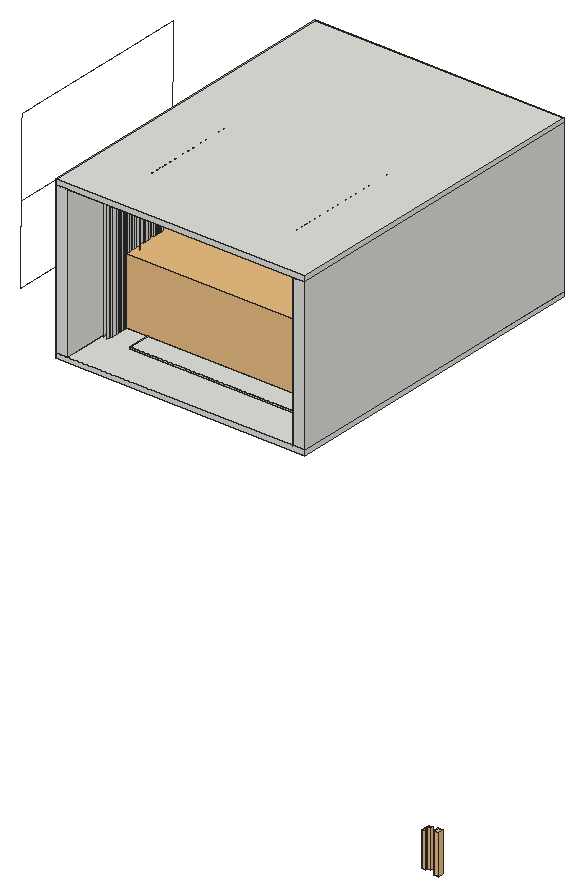
# SketchUp Ruby script. Lengths in millimetres.
U = 1.mm
M = Sketchup.active_model
def pt(a) = Geom::Point3d.new(a.map { |v| v * U })
def face(e, loops, mat)
  f = e.add_face(loops[0].map { |a| pt(a) })
  loops[1..].each { |l| e.add_face(l.map { |a| pt(a) }).erase! }
  f.material = f.back_material = mat if mat
  f
end
# faces: each face lists its corners as indices into pts; further lists are holes
def faces(e, pts, list, mat = nil) = list.each { |f| face(e, (f[0].is_a?(Array) ? f : [f]).map { |l| l.map { |i| pts[i] } }, mat) }
# xy, xz, yz: faces in a plane at the given z, y or x. An outline is a flat list of corners, or four numbers for a rectangle; further outlines are holes
def ring(l) = l.size == 4 ? [[l[0], l[1]], [l[2], l[1]], [l[2], l[3]], [l[0], l[3]]] : l.each_slice(2).to_a
def flat(e, list, mat, &to3) = list.each { |f| face(e, (f[0].is_a?(Array) ? f : [f]).map { |l| ring(l).map { |u, v| to3.(u, v) } }, mat) }
def xy(e, z, list, mat = nil) = flat(e, list, mat) { |x, y| [x, y, z] }
def xz(e, y, list, mat = nil) = flat(e, list, mat) { |x, z| [x, y, z] }
def yz(e, x, list, mat = nil) = flat(e, list, mat) { |y, z| [x, y, z] }
def lines(e, pts, list) = list.each { |a, b| e.add_line(pt(pts[a]), pt(pts[b])) }
# prism: a flat outline (further loops are holes) pulled along v
def prism(e, loops, v, mat = nil)
  f = face(e, loops, mat); d = Geom::Vector3d.new(v.map { |x| x * U })
  f.pushpull(f.normal.samedirection?(d) ? d.length : -d.length)
end
def box(e, o, s, mat = nil) = prism(e, [[o, [o[0] + s[0], o[1], o[2]], [o[0] + s[0], o[1] + s[1], o[2]], [o[0], o[1] + s[1], o[2]]]], [0, 0, s[2]], mat)
def at(x, y, z, deg = 0) = Geom::Transformation.translation(pt([x, y, z])) * Geom::Transformation.rotation(ORIGIN, Z_AXIS, deg.degrees)
def axes(o, x, y, z) = Geom::Transformation.new([*x, 0, *y, 0, *z, 0, *pt(o).to_a, 1])
def part(name) = M.definitions.add(name)
# library, detail: a bought-in or finely detailed component or shape, given as its bounding box
def library(name, o, s) = part(name).tap { |d| box(d.entities, o, s) }
def detail(e, o, s) = box(e.add_group.entities, o, s)
def put(e, d, t, mat = nil) = e.add_instance(d, t).tap { |i| i.material = mat if mat }
def group(e, t, mat = nil) = e.add_group.tap { |g| g.transformation = t; g.material = mat if mat }.entities
root = M.entities
M.materials.add("Glass").color = [171, 209, 242]
M.materials["Glass"].alpha = 0.1
M.materials.add("Plastic_SSS_01_White").color = [225, 221, 201]
M.materials.add("[0136_Charcoal]").color = [35, 35, 35]
M.materials.add("[Color A08]").color = [102, 0, 0]
M.materials.add("[Color M07]").color = [58, 58, 58]
M.materials.add("[Formica Beige]").color = [211, 187, 149]
M.materials.add("[Wood Veneer 01]").color = [120, 70, 37]
M.materials.add("тюль").color = [255, 255, 255]
M.materials["тюль"].alpha = 0.6
c1 = part("Area rug")
box(c1.entities,[0,0,0],[1400,2000,10])
c2 = part("Window frame")
xy(c2.entities,0,[[[2653.4,2133.1,4482.2,3352.3],[2704.2,2183.9,4431.4,3301.5]],[3237.6,2183.9,3288.4,3301.5],[3821.8,2183.9,3872.6,3301.5]],"Plastic_SSS_01_White")
xy(c2.entities,50.8,[[[2653.4,2133.1,4482.2,3352.3],[2704.2,2183.9,4431.4,3301.5]],[3237.6,2183.9,3288.4,3301.5],[3821.8,2183.9,3872.6,3301.5]],"Plastic_SSS_01_White")
xz(c2.entities,2133.1,[[2653.4,0,4482.2,50.8]],"Plastic_SSS_01_White")
xz(c2.entities,2183.9,[[2704.2,0,3237.6,50.8],[3237.6,0,3288.4,50.8],[3288.4,0,3821.8,50.8],[3821.8,0,3872.6,50.8],[3872.6,0,4431.4,50.8]],"Plastic_SSS_01_White")
xz(c2.entities,3301.5,[[2704.2,0,3237.6,50.8],[3237.6,0,3288.4,50.8],[3288.4,0,3821.8,50.8],[3821.8,0,3872.6,50.8],[3872.6,0,4431.4,50.8]],"Plastic_SSS_01_White")
xz(c2.entities,3352.3,[[2653.4,0,4482.2,50.8]],"Plastic_SSS_01_White")
yz(c2.entities,2653.4,[[2133.1,0,3352.3,50.8]],"Plastic_SSS_01_White")
yz(c2.entities,2704.2,[[2183.9,0,3301.5,50.8]],"Plastic_SSS_01_White")
yz(c2.entities,3237.6,[[2183.9,0,3301.5,50.8]],"Plastic_SSS_01_White")
yz(c2.entities,3288.4,[[2183.9,0,3301.5,50.8]],"Plastic_SSS_01_White")
yz(c2.entities,3821.8,[[2183.9,0,3301.5,50.8]],"Plastic_SSS_01_White")
yz(c2.entities,3872.6,[[2183.9,0,3301.5,50.8]],"Plastic_SSS_01_White")
yz(c2.entities,4431.4,[[2183.9,0,3301.5,50.8]],"Plastic_SSS_01_White")
yz(c2.entities,4482.2,[[2133.1,0,3352.3,50.8]],"Plastic_SSS_01_White")
c3 = part("Window glazing")
box(c3.entities,[0,0,0],[1724.1,1117.6,12.7])
c4 = part("Window assembly")
put(c4.entities,c2,at(-2653.4,-2133.1,0))
put(c4.entities,c3,at(50.8,50.8,17.8),"Glass")
c5 = part("window")
p = [[-15145.6,2238.1,518],[-16974.4,2238.1,518]]
lines(c5.entities,p,[[0,1]])
put(c5.entities,c4,axes([-16974.4,2238.1,518],[1,0,0],[0,0,1],[0,-1,0]))
c6 = part("Group\#61")
p = [[0,48,9.6],[0,48,40.8],[0,18.3,0],[0,0,25.2],[0,18.3,50.4]]
lines(c6.entities,p,[[0,1],[2,0],[3,2],[4,3],[1,4]])
c7 = part("Curtain panel")
yz(c7.entities,423.5,[[83.6,68.6,120.5,2032]])
p = [[42.2,57.1,68.6],[81.9,49.1,68.6],[81.9,49.1,2032],[42.2,57.1,2032],[89.6,60.6,68.6],[89.6,60.6,2032],
  [250.5,51.4,68.6],[262,49.4,68.6],[262,49.4,2032],[250.5,51.4,2032],[294,52.7,68.6],[294,52.7,2032],
  [234.4,66.2,68.6],[234.4,66.2,2032],[335.4,52.5,68.6],[351.9,52.1,68.6],[351.9,52.1,2032],[335.4,52.5,2032],
  [375.5,60,68.6],[375.5,60,2032],[332,60.7,68.6],[332,60.7,2032],[302.6,99.4,68.6],[302.6,99.4,2032],
  [113.7,56.1,68.6],[116.9,54,68.6],[116.9,54,2032],[113.7,56.1,2032],[130.3,54.1,68.6],[130.3,54.1,2032],
  [142.4,61.5,68.6],[142.4,61.5,2032],[485.4,55.1,68.6],[498.9,54.2,68.6],[498.9,54.2,2032],[485.4,55.1,2032],
  [509.2,55.8,2032],[509.2,55.8,68.6],[479.1,58.2,68.6],[479.1,58.2,2032],[168.4,60.1,68.6],[183.1,55.5,68.6],
  [183.1,55.5,2032],[168.4,60.1,2032],[205.8,56.2,68.6],[205.8,56.2,2032],[106,65.3,68.6],[106,65.3,2032],
  [220.7,98.3,68.6],[220.7,98.3,2032],[18.5,73.5,68.6],[18.5,73.5,2032],[475.8,65.4,68.6],[475.8,65.4,2032],
  [438.7,58.9,68.6],[448,58.5,68.6],[448,58.5,2032],[438.7,58.9,2032],[452.1,62.6,68.6],[452.1,62.6,2032],
  [428.3,61.4,68.6],[428.3,61.4,2032],[387.2,83.9,68.6],[387.2,83.9,2032],[165,66.8,68.6],[165,66.8,2032],
  [72.3,95.7,68.6],[72.3,95.7,2032],[343.3,92.9,68.6],[343.3,92.9,2032],[425,65.5,68.6],[425,65.5,2032],
  [156.5,93.7,68.6],[156.5,93.7,2032],[442.7,100.9,68.6],[442.7,100.9,2032],[100.8,87.1,68.6],[100.8,87.1,2032],
  [474.1,91.8,68.6],[474.1,91.8,2032],[423.5,83.6,68.6],[423.5,83.6,2032],[235.7,85.9,68.6],[235.7,85.9,2032],
  [190.8,117.3,68.6],[190.8,117.3,2032],[24.1,85.5,68.6],[24.1,85.5,2032],[379.7,124.4,68.6],[379.7,124.4,2032],
  [35.1,112.6,68.6],[35.1,112.6,2032],[267.2,131.4,68.6],[267.2,131.4,2032],[112,135,68.6],[112,135,2032],
  [486.8,123.6,68.6],[486.8,123.6,2032],[346.6,120.5,68.6],[346.6,120.5,2032],[152.9,128.5,68.6],[152.9,128.5,2032],
  [56.6,138.8,68.6],[56.6,138.8,2032],[221.5,129.5,68.6],[221.5,129.5,2032],[301.6,129,68.6],[301.6,129,2032],
  [432.5,131,68.6],[432.5,131,2032],[24,125.5,68.6],[24,125.5,2032],[173.3,137,68.6],[173.3,137,2032],
  [330.4,136,68.6],[330.4,136,2032],[409.6,134,68.6],[423.5,120.5,68.6],[423.5,120.5,2032],[409.6,134,2032],
  [473.8,143.8,68.6],[473.8,143.8,2032],[388.8,133.8,68.6],[388.8,133.8,2032],[0,139.4,68.6],[0,139.4,2032],
  [236.4,146.3,68.6],[236.4,146.3,2032],[439.5,142.5,2032],[439.5,142.5,68.6],[266.8,141.8,68.6],[266.8,141.8,2032],
  [101,147.4,68.6],[101,147.4,2032],[519.5,57.4,2032],[527.7,61.1,2032]]
faces(c7.entities,p,[[0,1,2,3],[1,4,5,2],[6,7,8,9],[7,10,11,8],[12,6,9,13],[14,15,16,17],[15,18,19,16],[20,14,17,21],
  [10,22,23,11],[24,25,26,27],[25,28,29,26],[28,30,31,29],[32,33,34,35],[36,34,33,37],[38,32,35,39],[40,41,42,43],
  [41,44,45,42],[46,24,27,47],[44,48,49,45],[50,0,3,51],[52,38,39,53],[54,55,56,57],[55,58,59,56],[60,54,57,61],
  [18,62,63,19],[64,40,43,65],[4,66,67,5],[68,20,21,69],[70,60,61,71],[30,72,73,31],[58,74,75,59],[76,46,47,77],
  [78,52,53,79],[80,70,71,81],[82,12,13,83],[84,64,65,85],[86,50,51,87],[62,88,89,63],[90,86,87,91],[92,82,83,93],
  [94,76,77,95],[96,78,79,97],[98,68,69,99],[72,100,101,73],[66,102,103,67],[48,104,105,49],[22,106,107,23],[74,108,109,75],
  [110,90,91,111],[112,84,85,113],[114,98,99,115],[116,117,118,119],[120,96,97,121],[88,122,123,89],[124,110,111,125],[100,112,113,101],
  [106,114,115,107],[104,126,127,105],[128,109,108,129],[130,92,93,131],[122,116,119,123],[132,94,95,133],[102,132,133,103],[126,130,131,127],
  [129,120,121,128]])
lines(c7.entities,p,[[134,135]])
put(c7.entities,c6,at(248.1,127.4,2032,-180))
put(c7.entities,c6,at(302.6,127.4,2032,-180))
put(c7.entities,c6,at(344,127.4,2032,-180))
put(c7.entities,c6,at(185.2,127.4,2032,-180))
put(c7.entities,c6,at(157,127.4,2032,-180))
put(c7.entities,c6,at(220.8,127.4,2032,-180))
put(c7.entities,c6,at(442.4,128,2032,-180))
put(c7.entities,c6,at(479,128,2032,-180))
put(c7.entities,c6,at(383.2,127.4,2032,-180))
put(c7.entities,c6,at(423.2,128,2032,-180))
put(c7.entities,c6,at(64.5,127.4,2032,-180))
put(c7.entities,c6,at(35.1,127.4,2032,-180))
put(c7.entities,c6,at(104.2,127.4,2032,-180))
c8 = part("end")
yz(c8.entities,0,[[32.5,25.8,24.5,28.4,24.5,36.8,32.5,39.4,37.5,32.6]])
p = [[50.8,0,12.5],[0,24.5,28.4],[0,32.5,25.8],[50.8,38.3,0],[101.6,13.8,21.4],[101.6,35.1,14.5],
  [0,37.5,32.6],[50.8,62,32.6],[101.6,48.2,32.6],[50.8,0,52.8],[0,24.5,36.8],[101.6,13.8,43.8],
  [0,32.5,39.4],[50.8,38.3,65.2],[101.6,35.1,50.7]]
faces(c8.entities,p,[[0,1,2,3],[4,0,3,5],[3,2,6,7],[3,7,8,5],[0,9,10,1],[4,11,9,0],[6,12,13,7],[7,13,14,8],
  [13,12,10,9],[14,13,9,11]])
c9 = part("Component\#75")
p = [[0,51.3,30.2],[0,25.7,48.8],[0,41.5,0],[0,0,30.2],[0,9.8,0]]
lines(c9.entities,p,[[0,1],[2,0],[3,4],[4,2],[1,3]])
c10 = part("Shower curtain\#1")
xy(c10.entities,-12.7,[[707,-12.7,2483.6,0]],"[0136_Charcoal]")
xy(c10.entities,0,[[707,-12.7,2483.6,0]],"[0136_Charcoal]")
xz(c10.entities,-12.7,[[707,-12.7,2483.6,0]],"[0136_Charcoal]")
xz(c10.entities,0,[[707,-12.7,2483.6,0]],"[0136_Charcoal]")
yz(c10.entities,707,[[-12.7,-12.7,0,0]])
yz(c10.entities,2483.6,[[-12.7,-12.7,0,0]],"[0136_Charcoal]")
put(c10.entities,c9,at(413.5,-33.6,-42.9))
put(c10.entities,c9,at(308,-33.6,-42.9))
put(c10.entities,c9,at(637.2,-33.6,-42.9))
put(c10.entities,c9,at(194.5,-33.6,-42.9))
put(c10.entities,c9,at(941,-33.6,-42.9))
put(c10.entities,c9,at(1223.4,-33.6,-42.9))
put(c10.entities,c9,at(761.7,-33.6,-42.9))
put(c10.entities,c9,at(875.2,-33.6,-42.9))
put(c10.entities,c9,at(1478.1,-33.6,-42.9))
put(c10.entities,c9,at(1328.9,-33.6,-42.9))
put(c10.entities,c9,at(81.1,-33.6,-42.9))
put(c10.entities,c9,at(534.9,-33.6,-42.9))
put(c10.entities,c9,at(1102,-33.6,-42.9))
g1 = group(c10.entities,at(18,-33,-2645.8))
p = [[684.3,109.4,0],[523.1,134.5,2.6],[523.1,25.1,2608.1],[684.3,0,2605.5],[803.4,168,6],[803.4,58.6,2611.6],
  [1212,109.4,0],[1177,123.4,1.4],[1177,14,2607],[1212,0,2605.5],[378.3,117.8,0.9],[322.3,156.9,4.9],
  [322.3,47.4,2610.4],[378.3,8.4,2606.4],[91.1,148.5,4],[0,123.4,1.4],[0,14,2607],[91.1,39.1,2609.6],
  [1153.7,148.5,4],[1153.7,39.1,2609.6],[175.2,126.2,1.7],[175.2,16.7,2607.3],[1008.9,131.7,2.3],[903.8,142.9,3.5],
  [903.8,33.5,2609],[1008.9,22.3,2607.8],[885.1,154.1,4.6],[885.1,44.7,2610.1]]
faces(g1,p,[[0,1,2,3],[4,0,3,5],[6,7,8,9],[10,11,12,13],[1,10,13,2],[14,15,16,17],[7,18,19,8],[20,14,17,21],
  [11,20,21,12],[22,23,24,25],[18,22,25,19],[23,26,27,24],[26,4,5,27]],"тюль")
g2 = group(c10.entities,at(1275.1,-33,-2645.8))
p = [[684.3,109.4,0],[523.1,134.5,2.6],[523.1,25.1,2608.1],[684.3,0,2605.5],[803.4,168,6],[803.4,58.6,2611.6],
  [1212,109.4,0],[1177,123.4,1.4],[1177,14,2607],[1212,0,2605.5],[378.3,117.8,0.9],[322.3,156.9,4.9],
  [322.3,47.4,2610.4],[378.3,8.4,2606.4],[91.1,148.5,4],[0,123.4,1.4],[0,14,2607],[91.1,39.1,2609.6],
  [1153.7,148.5,4],[1153.7,39.1,2609.6],[175.2,126.2,1.7],[175.2,16.7,2607.3],[1008.9,131.7,2.3],[903.8,142.9,3.5],
  [903.8,33.5,2609],[1008.9,22.3,2607.8],[885.1,154.1,4.6],[885.1,44.7,2610.1]]
faces(g2,p,[[0,1,2,3],[4,0,3,5],[6,7,8,9],[10,11,12,13],[1,10,13,2],[14,15,16,17],[7,18,19,8],[20,14,17,21],
  [11,20,21,12],[22,23,24,25],[18,22,25,19],[23,26,27,24],[26,4,5,27]],"тюль")
c11 = part("Группа\#112")
xy(c11.entities,34.5,[[707,9,2507,38]],"[0136_Charcoal]")
p = [[2507,23.5,0],[2507,0,13.2],[707,0,13.2],[707,23.5,0],[2507,47,13.2],[707,47,13.2],
  [2507,9,34.5],[707,9,34.5],[2507,38,34.5],[707,38,34.5]]
faces(c11.entities,p,[[0,1,2,3],[4,0,3,5],[1,6,7,2],[8,4,5,9]],"[0136_Charcoal]")
c12 = part("шторы раздвинутые\#1")
put(c12.entities,c7,axes([706.9,-2079.9,174.7],[1,0,0],[0,0,-0.36],[0,1,0]))
put(c12.entities,c7,axes([2242.4,-2079.9,174.7],[-1,0,0],[0,0,-0.36],[0,1,0]))
put(c12.entities,c8,axes([601.7,-53.1,137.5],[1,0,0],[0,0,-1],[0,1,0]),"[0136_Charcoal]")
put(c12.entities,c8,axes([2336.8,-53.1,137.5],[-1,0,0],[0,0,-1],[0,1,0]),"[0136_Charcoal]")
put(c12.entities,c10,axes([695.8,-38.1,43.6],[0.62018,0,0],[0,-0.03238,-0.99912],[0,0.7459,-0.04059]))
put(c12.entities,c11,axes([101.6,-38.6,89.2],[0.85105,0,0],[0,0.77173,0],[0,0,1]))
c13 = library("Кровать",[-199.4,-668.7,0],[2314.3,3237.4,1077.7])
c14 = part("Group103\#1")
p = [[0,0,0],[0,0,-1085.9],[-296.1,0,-1085.9],[1927.9,-1587.5,0],[-1927.9,-1587.5,0],[1927.9,1587.5,0],
  [1927.9,0,0],[-1927.9,1587.5,0],[296.1,0,-1085.9],[-1927.9,0,0],[0,0,-1757.7]]
lines(c14.entities,p,[[0,1],[1,2],[3,4],[5,6],[7,5],[1,8],[9,0],[0,6],[8,10],[4,9],[6,3],[2,10],
  [9,7]])
c15 = part("Rectangle Light")
put(c15.entities,c14,at(0,0,0))
c16 = library("Ceiling Lamp 298 001",[-202.8,-202.9,-2651.1],[405.4,405.9,2659.1])
c17 = library("Wardrobe 27-03",[-1541,-325,0],[3082,650,2384])
c18 = library("Group\#27",[0,0,0],[75,66,697.2])
c19 = library("Group\#25",[7.6,7.6,18.4],[67.4,50.8,763.8])
c20 = library("Group\#28",[-17,-17,-14.7],[100,100,796.9])
c21 = library("Group\#29",[-12.7,-12.7,0],[584.2,25.4,558.8])
c22 = library("Group\#32",[-12.7,-12.7,0],[2939.6,4463.6,76.2])
put(root,c1,axes([838.2,829.6,25.4],[2.39,0,0],[0,2.74751,0],[0,0,1]))
put(root,c5,axes([-9843.1,-24134.9,113],[0,-1.68056,0],[4.5,0,0],[0,0,1.4375]))
put(root,c12,axes([228.6,-1100.1,2857.6],[0,2.738,0],[0,0,1.41753],[1,0,0]))
put(root,c13,axes([1100.6,5506.8,35.4],[0,-2,0],[1.4404,0,0],[0,0,1.24]))
put(root,c15,axes([-1512,2920.2,1782.1],[0.00427,-0.99999,0.00252],[-0.00823,-0.00256,-0.99996],[-0.99996,-0.00425,0.00824]))
put(root,c16,axes([3720.9,5917.6,2984.4],[0.4224,0,0],[0,0.39,0],[0,0,0.35037]))
put(root,c16,axes([4010.1,5917.6,2984.4],[0.4224,0,0],[0,0.39,0],[0,0,0.35037]))
put(root,c16,axes([704.8,5917.6,2984.4],[0.4224,0,0],[0,0.39,0],[0,0,0.35037]))
put(root,c16,axes([994,5917.6,2984.4],[0.4224,0,0],[0,0.39,0],[0,0,0.35037]))
put(root,c17,axes([4592.6,2336.8,344.2],[0,-1,0],[0.64,0,0],[0,0,1]))
g3 = group(root,at(0,0,0))
xy(g3,0,[[0,0,228.6,6553.2]])
xy(g3,857.6,[[0,1318.2,228.6,4391.6]])
xy(g3,2610.2,[[0,1318.2,228.6,4391.6]])
xy(g3,3048,[[0,0,228.6,6553.2]])
xz(g3,0,[[0,0,228.6,3048]])
xz(g3,1318.2,[[0,857.6,228.6,2610.2]])
xz(g3,4391.6,[[0,857.6,228.6,2610.2]])
xz(g3,6553.2,[[0,0,228.6,3048]])
yz(g3,0,[[[0,0,6553.2,3048],[1318.2,857.6,4391.6,2610.2]]])
yz(g3,228.6,[[[0,0,6324.6,3048],[1318.2,857.6,4391.6,2610.2]],[6324.6,0,6553.2,3048]])
g4 = group(root,at(228.6,6324.6,0))
xy(g4,0,[[0,0,0,228.6,4572,228.6,4572,0,2272,0,2272,12.7,2259.3,12.7,2259.3,0,2219.6,0,2219.6,12.7,2206.9,12.7,2206.9,0,2167.1,0,2167.1,12.7,2154.4,12.7,2154.4,0,1851.3,0,1851.3,12.7,1838.6,12.7,1838.6,0,1798.8,0,1798.8,12.7,1786.1,12.7,1786.1,0,1746.4,0,1746.4,12.7,1733.7,12.7,1733.7,0,1694,0,1694,12.7,1681.3,12.7,1681.3,0,1641.6,0,1641.6,12.7,1628.9,12.7,1628.9,0,1589.1,0,1589.1,12.7,1576.4,12.7,1576.4,0,1536.8,0,1536.8,12.7,1524,12.7,1524,0]])
xy(g4,3048,[[0,0,1524,0,1524,12.7,1536.8,12.7,1536.8,0,1576.4,0,1576.4,12.7,1589.1,12.7,1589.1,0,1628.9,0,1628.9,12.7,1641.6,12.7,1641.6,0,1681.3,0,1681.3,12.7,1694,12.7,1694,0,1733.7,0,1733.7,12.7,1746.4,12.7,1746.4,0,1786.1,0,1786.1,12.7,1798.8,12.7,1798.8,0,1838.6,0,1838.6,12.7,1851.3,12.7,1851.3,0,2154.4,0,2154.4,12.7,2167.1,12.7,2167.1,0,2206.9,0,2206.9,12.7,2219.6,12.7,2219.6,0,2259.3,0,2259.3,12.7,2272,12.7,2272,0,4572,0,4572,228.6,0,228.6]])
xz(g4,0,[[2803,0,3048,3048]],"[Color M07]")
xz(g4,0,[[1536.8,0,1576.4,3048],[1589.1,0,1628.9,3048],[1641.6,0,1681.3,3048],[1694,0,1733.7,3048],[1746.4,0,1786.1,3048],
  [1798.8,0,1838.6,3048],[1851.3,0,2154.4,3048],[2167.1,0,2206.9,3048],[2219.6,0,2259.3,3048],[2272,0,2803,3048],
  [3048,0,4572,3048]],"[Formica Beige]")
xz(g4,0,[[0,0,1524,3048]],"[Wood Veneer 01]")
xz(g4,12.7,[[1524,0,1536.8,3048],[1576.4,0,1589.1,3048],[1628.9,0,1641.6,3048],[1681.3,0,1694,3048],[1733.7,0,1746.4,3048],
  [1786.1,0,1798.8,3048],[1838.6,0,1851.3,3048],[2154.4,0,2167.1,3048],[2206.9,0,2219.6,3048],[2259.3,0,2272,3048]],"[Color M07]")
xz(g4,228.6,[[0,0,4572,3048]])
yz(g4,0,[[0,0,228.6,3048]])
yz(g4,1524,[[0,0,12.7,3048]],"[Color M07]")
yz(g4,1536.8,[[0,0,12.7,3048]],"[Color M07]")
yz(g4,1576.4,[[0,0,12.7,3048]],"[Color M07]")
yz(g4,1589.1,[[0,0,12.7,3048]],"[Color M07]")
yz(g4,1628.9,[[0,0,12.7,3048]],"[Color M07]")
yz(g4,1641.6,[[0,0,12.7,3048]],"[Color M07]")
yz(g4,1681.3,[[0,0,12.7,3048]],"[Color M07]")
yz(g4,1694,[[0,0,12.7,3048]],"[Color M07]")
yz(g4,1733.7,[[0,0,12.7,3048]],"[Color M07]")
yz(g4,1746.4,[[0,0,12.7,3048]],"[Color M07]")
yz(g4,1786.1,[[0,0,12.7,3048]],"[Color M07]")
yz(g4,1798.8,[[0,0,12.7,3048]],"[Color M07]")
yz(g4,1838.6,[[0,0,12.7,3048]],"[Color M07]")
yz(g4,1851.3,[[0,0,12.7,3048]],"[Color M07]")
yz(g4,2154.4,[[0,0,12.7,3048]],"[Color M07]")
yz(g4,2167.1,[[0,0,12.7,3048]],"[Color M07]")
yz(g4,2206.9,[[0,0,12.7,3048]],"[Color M07]")
yz(g4,2219.6,[[0,0,12.7,3048]],"[Color M07]")
yz(g4,2259.3,[[0,0,12.7,3048]],"[Color M07]")
yz(g4,2272,[[0,0,12.7,3048]],"[Color M07]")
yz(g4,4572,[[0,0,228.6,3048]])
g5 = group(root,at(4800.6,0,0))
prism(g5,[[[0,0,0],[0,6324.6,0],[0,6553.2,0],[228.6,6553.2,0],[228.6,0,0]]],[0,0,3048])
g6 = group(root,at(0,0,-101.6))
xy(g6,0,[[[0,0,5029.2,6553.2],[228.6,228.6,4800.6,6324.6]],[228.6,228.6,4800.6,6324.6]])
xy(g6,101.6,[[0,0,5029.2,6553.2]])
xz(g6,0,[[0,0,5029.2,101.6]])
xz(g6,6324.6,[[228.6,0,4800.6,101.6]])
xz(g6,6553.2,[[0,0,5029.2,101.6]])
yz(g6,0,[[0,0,6553.2,101.6]])
yz(g6,228.6,[[228.6,0,6324.6,101.6]])
yz(g6,4800.6,[[228.6,0,6324.6,101.6]])
yz(g6,5029.2,[[0,0,6553.2,101.6]])
g7 = group(root,at(838.2,829.6,0))
box(g7,[0,0,0],[3352.8,5495,25.4])
put(root,c18,at(15026.1,-9526.1,108.3))
put(root,c19,at(15119.1,-9526.1,108.3))
put(root,c20,at(15305.1,-9526.1,108.3))
g8 = group(root,at(2121.7,6299.2,1899))
prism(g8,[[[351.6,25.4,91.4],[340.5,25.4,75],[327.7,25.4,59.9],[313.4,25.4,46.1],[297.7,25.4,33.9],[280.9,25.4,23.5],[263,25.4,14.8],[244.4,25.4,8.1],[225.1,25.4,3.4],[205.5,25.4,0.6],[185.6,25.4,0],[165.9,25.4,1.4],[146.3,25.4,4.9],[127.3,25.4,10.4],[108.9,25.4,17.9],[91.4,25.4,27.3],[75,25.4,38.4],[59.9,25.4,51.2],[46.1,25.4,65.5],[33.9,25.4,81.2],[23.5,25.4,98],[14.8,25.4,115.9],[8.1,25.4,134.5],[3.4,25.4,153.8],[0.6,25.4,173.4],[0,25.4,193.2],[1.4,25.4,213],[4.9,25.4,232.5],[10.4,25.4,251.6],[17.9,25.4,270],[27.3,25.4,287.4],[38.4,25.4,303.9],[51.2,25.4,319],[65.5,25.4,332.8],[81.2,25.4,344.9],[98,25.4,355.4],[115.9,25.4,364],[134.5,25.4,370.8],[153.8,25.4,375.5],[173.4,25.4,378.2],[193.2,25.4,378.9],[213,25.4,377.4],[232.5,25.4,373.9],[251.6,25.4,368.4],[270,25.4,361],[287.4,25.4,351.6],[303.9,25.4,340.5],[319,25.4,327.7],[332.8,25.4,313.4],[344.9,25.4,297.7],[355.4,25.4,280.9],[364,25.4,263],[370.8,25.4,244.4],[375.5,25.4,225.1],[378.2,25.4,205.5],[378.9,25.4,185.6],[377.4,25.4,165.9],[373.9,25.4,146.3],[368.4,25.4,127.3],[361,25.4,108.9]]],[0,-25.4,0])
put(root,c21,at(1842.3,6248.4,1812.9))
g9 = group(root,at(0,0,3048))
xy(g9,0,[[[0,0,5029.2,6553.2],[966.3,966.3,4062.9,5586.9]]])
xy(g9,0,[[[966.3,966.3,4062.9,5586.9],[1057.5,1057.5,3971.7,5495.7]]],"[Color A08]")
xy(g9,76.2,[[1057.5,1057.5,3971.7,5495.7]])
xy(g9,101.6,[[0,0,5029.2,6553.2]])
xz(g9,0,[[0,0,5029.2,101.6]])
xz(g9,1057.5,[[1057.5,0,3971.7,76.2]])
xz(g9,5495.7,[[1057.5,0,3971.7,76.2]])
xz(g9,6553.2,[[0,0,5029.2,101.6]])
yz(g9,0,[[0,0,6553.2,101.6]])
yz(g9,1057.5,[[1057.5,0,5495.7,76.2]])
yz(g9,3971.7,[[1057.5,0,5495.7,76.2]])
yz(g9,5029.2,[[0,0,6553.2,101.6]])
put(root,c22,at(1057.5,1057.5,3048))
